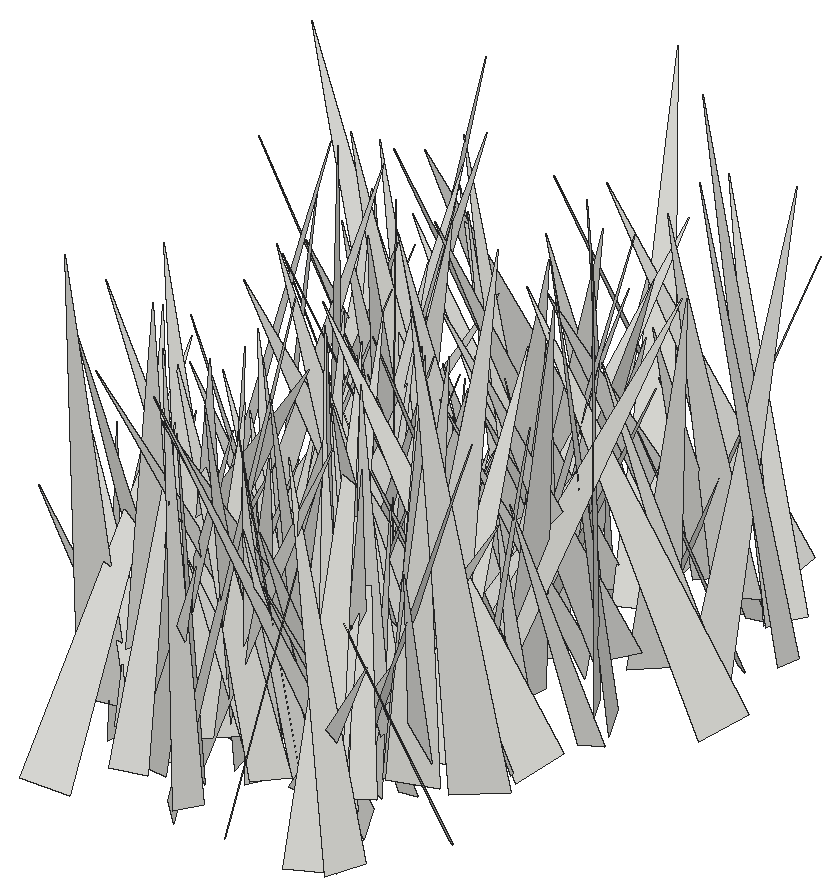
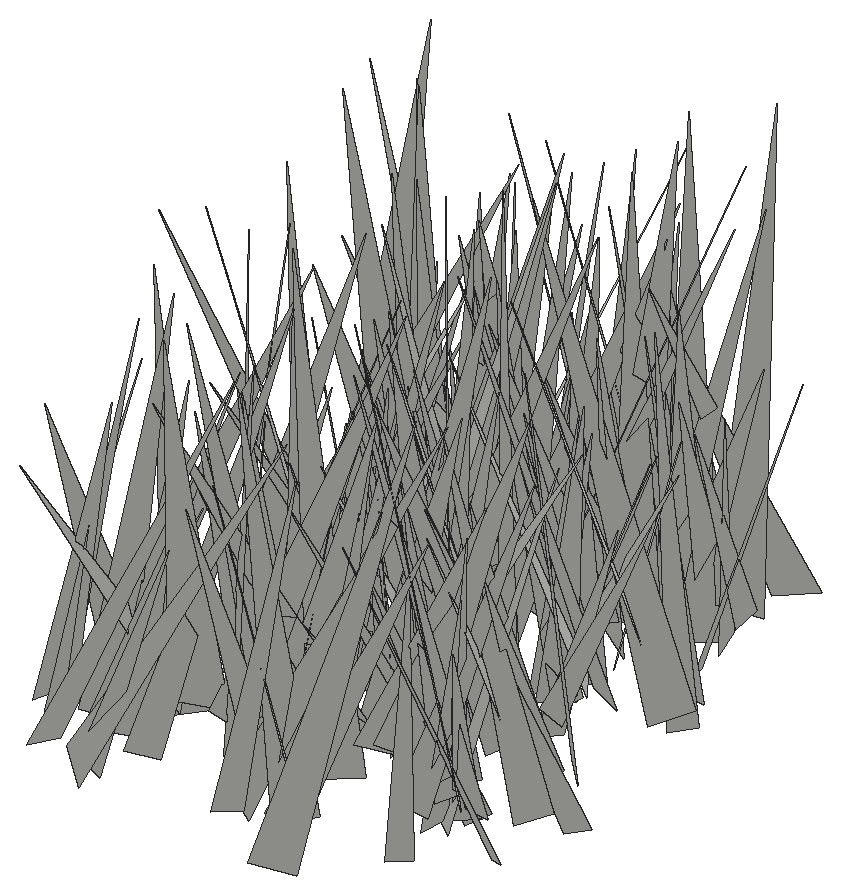
# SketchUp Ruby script. Lengths in inches.
U = 1.inch
M = Sketchup.active_model
def pt(a) = Geom::Point3d.new(a.map { |v| v * U })
def face(e, loops, mat)
  f = e.add_face(loops[0].map { |a| pt(a) })
  loops[1..].each { |l| e.add_face(l.map { |a| pt(a) }).erase! }
  f.material = f.back_material = mat if mat
  f
end
# faces: each face lists its corners as indices into pts; further lists are holes
def faces(e, pts, list, mat = nil) = list.each { |f| face(e, (f[0].is_a?(Array) ? f : [f]).map { |l| l.map { |i| pts[i] } }, mat) }
# xy, xz, yz: faces in a plane at the given z, y or x. An outline is a flat list of corners, or four numbers for a rectangle; further outlines are holes
def ring(l) = l.size == 4 ? [[l[0], l[1]], [l[2], l[1]], [l[2], l[3]], [l[0], l[3]]] : l.each_slice(2).to_a
def flat(e, list, mat, &to3) = list.each { |f| face(e, (f[0].is_a?(Array) ? f : [f]).map { |l| ring(l).map { |u, v| to3.(u, v) } }, mat) }
def xy(e, z, list, mat = nil) = flat(e, list, mat) { |x, y| [x, y, z] }
def xz(e, y, list, mat = nil) = flat(e, list, mat) { |x, z| [x, y, z] }
def yz(e, x, list, mat = nil) = flat(e, list, mat) { |y, z| [x, y, z] }
def lines(e, pts, list) = list.each { |a, b| e.add_line(pt(pts[a]), pt(pts[b])) }
# prism: a flat outline (further loops are holes) pulled along v
def prism(e, loops, v, mat = nil)
  f = face(e, loops, mat); d = Geom::Vector3d.new(v.map { |x| x * U })
  f.pushpull(f.normal.samedirection?(d) ? d.length : -d.length)
end
def box(e, o, s, mat = nil) = prism(e, [[o, [o[0] + s[0], o[1], o[2]], [o[0] + s[0], o[1] + s[1], o[2]], [o[0], o[1] + s[1], o[2]]]], [0, 0, s[2]], mat)
def at(x, y, z, deg = 0) = Geom::Transformation.translation(pt([x, y, z])) * Geom::Transformation.rotation(ORIGIN, Z_AXIS, deg.degrees)
def axes(o, x, y, z) = Geom::Transformation.new([*x, 0, *y, 0, *z, 0, *pt(o).to_a, 1])
def part(name) = M.definitions.add(name)
# library, detail: a bought-in or finely detailed component or shape, given as its bounding box
def library(name, o, s) = part(name).tap { |d| box(d.entities, o, s) }
def detail(e, o, s) = box(e.add_group.entities, o, s)
def put(e, d, t, mat = nil) = e.add_instance(d, t).tap { |i| i.material = mat if mat }
def group(e, t, mat = nil) = e.add_group.tap { |g| g.transformation = t; g.material = mat if mat }.entities
root = M.entities
c1 = part("fur_instance\#9")
p = [[0.8125,0,1.79],[0.67,-0.02,1.48],[0,-0.11,0],[0,0.11,0]]
faces(c1.entities,p,[[0,1,2,3]])
put(root,c1,axes([114.02,116.04,-27.1],[-0.24742,-3.68689,1.2628],[-3.55064,-0.30834,-1.59591],[-1.60648,1.24932,3.33279]))
put(root,c1,axes([111.5,119.83,-27.1],[4.04394,2.43918,0.42992],[2.39305,-4.06014,0.52577],[-0.63852,0.23141,4.69325]))
put(root,c1,axes([113.03,117.41,-28.22],[-4.3486,2.21974,0.80785],[1.83051,4.23636,-1.78683],[1.49303,1.27131,4.54366]))
put(root,c1,axes([113.39,120.65,-28.22],[-2.57238,2.98987,0.10946],[2.97729,2.57237,-0.29516],[0.29502,0.10983,3.93311]))
put(root,c1,axes([115.94,120.41,-27.1],[-4.22364,6.9226,0.63988],[6.72709,3.88063,2.42031],[-1.75445,-1.78585,7.73974]))
put(root,c1,axes([110.48,119.21,-28.22],[0.87918,5.14411,1.43079],[4.85097,-0.16366,-2.39235],[2.23095,-1.67133,4.63805]))
put(root,c1,axes([110.67,121.02,-27.1],[5.28357,-2.5058,0.04843],[-2.504,-5.27298,0.35108],[0.10676,0.33794,5.83712]))
put(root,c1,axes([113.7,121.4,-28.22],[-3.65311,-4.50937,0.62916],[-4.48426,3.70309,0.50402],[0.78847,0.16789,5.78149]))
put(root,c1,axes([113.92,121.53,-28.22],[-4.36363,0.98227,0.81119],[0.91976,4.432,-0.41906],[0.88144,0.23814,4.45315]))
put(root,c1,axes([113.81,122.78,-27.1],[0.77993,-5.26102,0.56712],[-5.12867,-0.89269,-1.22806],[-1.30258,0.36472,5.1748]))
put(root,c1,axes([114.15,120.3125,-27.1],[-5.02502,0.15502,0.9974],[-0.08895,4.97687,-1.22169],[1.00545,1.21508,4.87671]))
put(root,c1,axes([113.62,109.8,-28.22],[-4.09527,-2.1175,0.66115],[-1.87882,4.04889,1.32991],[1.17939,-0.90267,4.41434]))
put(root,c1,axes([113.2,108.08,-27.1],[-3.70619,1.07071,1.22273],[0.63141,3.75399,-1.37341],[1.4976,1.06701,3.605]))
put(root,c1,axes([112.73,116.55,-28.22],[4.54729,4.68314,2.12923],[4.88324,-4.82336,0.17985],[-1.61844,-1.39522,6.52513]))
put(root,c1,axes([114.97,115.28,-28.22],[-4.74174,-2.50609,0.51828],[-2.55748,4.67952,-0.77105],[0.09149,0.92453,5.30754]))
put(root,c1,axes([114.01,107.99,-28.22],[-4.48133,-0.60292,1.35721],[-0.97091,4.45413,-1.22715],[1.12377,1.44397,4.35201]))
put(root,c1,axes([114.64,115.36,-28.22],[-3.82314,1.91513,0.41484],[1.95484,3.79049,0.51675],[0.13566,-0.64863,4.24466]))
put(root,c1,axes([114.16,116.82,-28.22],[-5.42402,3.35952,0.54018],[3.08821,5.28712,-1.87283],[1.42868,1.32596,6.09909]))
put(root,c1,axes([116.91,119.8,-27.1],[-5.49378,-4.48735,0.1731],[-4.21573,5.05933,-2.64174],[-1.54724,2.14821,6.58325]))
put(root,c1,axes([111.83,112.71,-28.22],[5.73315,-1.08828,0.33068],[-0.98004,-5.58896,-1.40205],[-0.57725,-1.3198,5.66459]))
put(root,c1,axes([115.26,107.1,-27.1],[-5.60466,1.1961,0.32776],[0.92969,5.05609,-2.5538],[0.82084,2.4404,5.13039]))
put(root,c1,axes([111.19,122.08,-28.22],[3.29682,4.04593,0.27696],[3.82738,-2.98619,-1.93627],[1.34069,-1.42422,4.84659]))
put(root,c1,axes([115.87,107.25,-27.1],[-2.49681,4.68547,0.3153],[4.52882,2.308,1.56527],[-1.24213,-1.0033,5.07323]))
put(root,c1,axes([113.27,112.22,-27.1],[5.00071,5.94343,0.88428],[5.7504,-5.06729,1.53914],[-1.74336,0.3341,7.61331]))
put(root,c1,axes([113.77,107.82,-27.1],[1.30407,-7.61557,2.3618],[-7.95747,-1.39423,-0.10194],[-0.50366,2.30972,7.72574]))
put(root,c1,axes([114.55,112.42,-27.1],[-3.02688,-2.08558,0.64094],[-2.07151,3.09116,0.27563],[0.68504,0.13224,3.66547]))
put(root,c1,axes([115.68,113.24,-27.1],[-2.7303,-2.91554,0.15676],[-2.8364,2.59761,-1.08937],[-0.69267,0.85529,3.84294]))
put(root,c1,axes([116.74,120.65,-27.1],[-3.94655,4.7323,0.06828],[4.56087,3.77904,1.70056],[-1.26405,-1.13963,5.92267]))
put(root,c1,axes([112.63,111.09,-28.22],[-1.89095,-4.65132,2.366],[-4.60338,2.67208,1.57395],[2.45798,1.42605,4.76793]))
put(root,c1,axes([112.15,121.8,-27.1],[3.4737,5.90005,1.74495],[6.11319,-3.08303,-1.74525],[0.69596,-2.36778,6.62052]))
put(root,c1,axes([113.4,123.78,-28.22],[3.7269,-2.05729,0.24824],[-1.97365,-3.67974,-0.86491],[-0.63149,-0.64103,4.16823]))
put(root,c1,axes([113.13,121.38,-27.1],[5.7382,5.20942,1.87337],[5.41352,-5.84467,-0.3291],[-1.15821,-1.50876,7.74318]))
put(root,c1,axes([113.33,121.5625,-27.1],[4.73571,-1.08461,0.9225],[-1.0987,-4.82145,-0.02851],[-0.90568,0.17765,4.85824]))
put(root,c1,axes([114.72,127.98,-27.1],[4.75153,-4.99406,0.9078],[-4.47168,-4.70683,-2.48828],[-2.40183,-1.11663,6.42854]))
put(root,c1,axes([115.76,107.52,-28.22],[-5.08982,4.44528,0.70369],[4.40622,5.13821,-0.58816],[0.91699,-0.01575,6.73207]))
put(root,c1,axes([112.84,111.25,-28.22],[4.26787,-0.90452,0.30078],[-0.95208,-4.11231,1.14272],[-0.04649,1.18073,4.21035]))
put(root,c1,axes([115.4375,109.34,-27.1],[-1.29627,-6.42722,1.30707],[-6.54569,1.18361,-0.67151],[-0.41416,1.4099,6.52216]))
put(root,c1,axes([115.58,114.3,-28.22],[-4.07009,-1.55263,0.42821],[-1.43545,4.0247,0.94922],[0.73043,-0.7422,4.25151]))
put(root,c1,axes([114.27,104.43,-28.22],[-2.48989,6.58556,0.19317],[6.42005,2.47161,-1.51018],[1.47984,0.3578,6.87667]))
put(root,c1,axes([115.29,120.33,-28.22],[0.65749,-6.30029,1.7132],[-6.47052,-0.85883,-0.67511],[-0.87239,1.62165,6.29842]))
put(root,c1,axes([113.45,114.24,-27.1],[3.5873,6.66463,1.07182],[6.75002,-3.55215,-0.50434],[-0.05834,-1.18311,7.55193]))
put(root,c1,axes([115.72,113.67,-28.22],[3.17127,-3.30736,3.04126],[-3.82504,-3.9403,-0.2965],[-2.35731,1.94429,4.57249]))
put(root,c1,axes([113.14,120.47,-28.22],[2.74116,-2.85153,0.16279],[-2.64199,-2.44575,1.64616],[1.08517,1.2485,3.59657]))
put(root,c1,axes([117.54,123.87,-28.22],[-4.20776,3.77593,1.0344],[3.85861,3.7428,2.0336],[-0.66241,-2.18328,5.27517]))
put(root,c1,axes([113.4,118.2,-27.1],[4.3525,2.53578,0.43229],[2.57081,-4.2585,-0.90411],[0.08934,-0.99816,4.9555]))
put(root,c1,axes([115.15,116.42,-28.22],[-5.30404,4.85737,1.41696],[4.30663,5.41145,-2.42976],[2.65607,0.92563,6.76928]))
put(root,c1,axes([111.27,113.91,-27.1],[2.01455,-7.63294,0.11302],[-6.59973,-1.68273,3.99311],[3.83642,1.11337,6.80994]))
put(root,c1,axes([116.54,113.45,-28.22],[-5.03296,-0.41167,1.23228],[-0.52474,5.15421,-0.42127],[1.18855,0.5323,5.03216]))
put(root,c1,axes([116.49,113.04,-28.22],[-3.50037,2.65675,1.28484],[2.86731,3.53339,0.50538],[0.69832,-1.19104,4.36526]))
put(root,c1,axes([114.875,108.5,-28.22],[4.71718,-6.41333,2.08506],[-6.64537,-4.85367,0.10513],[-1.14777,1.74389,7.96063]))
put(root,c1,axes([116.49,110.02,-28.22],[2.34142,5.16985,1.64131],[5.10687,-2.70355,1.23051],[-1.82787,-0.93109,5.54034]))
put(root,c1,axes([114.38,113.92,-27.1],[4.71146,3.59222,0.48874],[3.58656,-4.73541,0.23065],[-0.52868,-0.11206,5.92019]))
put(root,c1,axes([119.03,108.63,-27.1],[-7.40149,0.22253,0.007],[0.22253,7.40149,0.00759],[0.00677,-0.0078,7.40483]))
put(root,c1,axes([115.52,108.19,-28.22],[4.65785,-0.69082,1.21899],[-0.53967,-4.78978,-0.65231],[-1.29303,-0.48941,4.6634]))
put(root,c1,axes([119.43,116.89,-28.22],[-0.98442,7.82804,0.7856],[7.24103,0.59195,3.17514],[-3.07617,-1.11168,7.22258]))
put(root,c1,axes([119.22,123.96,-28.22],[-3.5976,-6.50533,0.64098],[-6.34012,3.29439,-2.15004],[-1.59153,1.58132,7.11613]))
put(root,c1,axes([117.55,108.19,-27.1],[3.71191,-5.65782,4.04126],[-6.28277,-4.69165,-0.79764],[-2.97818,2.84578,6.7196]))
put(root,c1,axes([118.01,118.71,-28.22],[-4.3642,6.37446,3.0679],[7.06974,4.05938,1.62241],[0.25406,-3.46117,7.553]))
put(root,c1,axes([116.57,109.33,-27.1],[-1.7521,4.37342,1.24469],[4.49457,1.86786,-0.23622],[0.6891,-1.06311,4.7054]))
put(root,c1,axes([116.49,114.98,-27.1],[7.01213,2.59998,3.36264],[2.81322,-7.70163,0.08845],[-3.18638,-1.07803,7.47811]))
put(root,c1,axes([115.33,113.61,-28.22],[4.85484,-0.93426,0.93937],[-1.01134,-4.91828,0.33525],[-0.85583,0.51221,4.93253]))
put(root,c1,axes([119.17,120.8,-28.22],[-6.47288,0.26814,0.01301],[0.25719,6.28405,-1.55397],[0.07694,1.55212,6.2893]))
put(root,c1,axes([116.85,105.0625,-27.1],[-1.85743,4.94831,0.92273],[4.99711,1.93095,-0.29602],[0.60509,-0.75691,5.27714]))
put(root,c1,axes([115.04,119.2,-28.22],[4.2743,-5.66959,1.70794],[-5.91958,-4.14155,1.06631],[-0.14077,2.00854,7.01974]))
put(root,c1,axes([116.39,111.77,-27.1],[-0.0874,4.08723,0.80677],[4.1529,0.14964,-0.30818],[0.33125,-0.79758,4.07653]))
put(root,c1,axes([115.93,115.375,-28.22],[5.15399,5.0376,1.12923],[4.93282,-5.27609,1.02292],[-1.5231,-0.04087,7.13405]))
put(root,c1,axes([115.65,110.125,-27.1],[5.14782,-4.26055,1.16689],[-4.27581,-5.25589,-0.32723],[-1.10966,0.4872,6.67423]))
put(root,c1,axes([115.52,119.42,-28.22],[7.57168,-2.77915,1.4038],[-2.39268,-7.55557,-2.05259],[-1.99233,-1.48808,7.80006]))
put(root,c1,axes([116.4,115.59,-27.1],[-0.03084,5.75903,1.17934],[5.85206,0.14189,-0.53988],[0.55736,-1.17118,5.73375]))
put(root,c1,axes([118.19,111.2,-27.1],[-6.16351,-3.9605,0.27898],[-3.73191,5.95492,2.08903],[1.35509,-1.6142,7.02213]))
put(root,c1,axes([116.01,109.52,-27.1],[4.17653,-0.25853,0.87813],[-0.4857,-4.1025,1.10224],[-0.77592,1.17643,4.03674]))
put(root,c1,axes([114.96,109.01,-27.1],[3.94876,4.2171,2.00571],[4.64379,-3.26946,-2.26834],[0.4919,-2.98768,5.31331]))
put(root,c1,axes([117.28,107.8,-28.22],[-3.42106,-4.15596,2.05732],[-4.44833,3.66341,0.00339],[1.31032,1.58608,5.3829]))
put(root,c1,axes([115.7,112.32,-28.22],[4.00821,-3.73033,0.31245],[-3.73197,-4.01777,-0.09299],[-0.29215,0.14465,5.47471]))
put(root,c1,axes([116.73,116.02,-28.22],[-0.99114,4.85366,1.48422],[5.00835,1.18049,-0.51592],[0.82303,-1.33855,4.92689]))
put(root,c1,axes([118.53,120.74,-27.1],[-5.56537,0.35389,1.01892],[0.25962,5.63719,-0.53984],[1.04691,0.48332,5.55042]))
put(root,c1,axes([118.12,112.79,-28.22],[0.5097,3.85536,0.87755],[3.83119,-0.70034,0.85159],[-0.9777,-0.73445,3.79452]))
put(root,c1,axes([118.95,116.91,-28.22],[-7.12654,1.94071,2.81889],[3.04033,6.57978,3.15641],[1.57127,-3.9294,6.67765]))
put(root,c1,axes([116.65,110.62,-27.1],[5.33264,0.16428,1.51785],[-0.27785,-5.31816,1.55174],[-1.50122,1.56784,5.10452]))
put(root,c1,axes([115.97,107.14,-28.22],[1.4923,-4.43759,0.64343],[-4.35505,-1.27294,1.3215],[1.06759,1.01025,4.49142]))
put(root,c1,axes([119.5,104.49,-27.1],[-6.71,0.21588,0.88951],[-0.0468,6.49159,-1.92847],[0.91413,1.91692,6.43053]))
put(root,c1,axes([116.26,116.11,-27.1],[4.91416,0.05831,0.74386],[0.02898,-4.96646,0.19783],[-0.74558,0.19125,4.91052]))
put(root,c1,axes([117.86,126.13,-27.1],[-4.50462,1.14541,2.32905],[1.86637,4.67145,1.31236],[1.80364,-1.97324,4.45884]))
put(root,c1,axes([117.9,118.83,-27.1],[-4.53794,-6.8341,0.16977],[-6.57814,4.42074,2.12406],[1.86058,-1.03861,7.92377]))
put(root,c1,axes([119.57,115.48,-28.22],[-5.44212,1.96061,0.21811],[1.90755,5.39324,-0.88463],[0.50284,0.7598,5.71648]))
put(root,c1,axes([120.79,119.32,-28.22],[-0.71343,7.62578,1.29035],[7.14993,0.15622,3.02994],[-2.94889,-1.46615,7.03427]))
put(root,c1,axes([116.5,118.18,-28.22],[1.15422,4.7345,0.08294],[4.6056,-1.10261,-1.15208],[1.10037,-0.35121,4.73502]))
put(root,c1,axes([119.75,123.21,-28.22],[-5.4355,-1.48683,0.1699],[-1.41481,5.31415,1.24191],[0.48767,-1.15472,5.49664]))
put(root,c1,axes([117.7,118.57,-28.22],[3.13173,2.6382,1.54856],[2.8558,-3.31576,-0.12654],[-1.0966,-1.10068,4.0929]))
put(root,c1,axes([120.31,107.28,-27.1],[-1.88222,6.06948,1.49765],[6.0067,1.32242,2.18977],[-1.73238,-2.00921,5.96542]))
put(root,c1,axes([119.08,112.77,-28.22],[2.70234,-6.75975,0.1599],[-6.39067,-2.60962,-2.31767],[-2.20886,-0.71979,6.90111]))
put(root,c1,axes([117.62,109.67,-28.22],[6.82649,-0.20783,2.36031],[0.47416,-6.93274,-1.9818],[-2.32152,-2.02711,6.5358]))
put(root,c1,axes([116.67,124.43,-27.1],[3.8282,2.91024,0.83789],[3.01788,-3.55309,-1.44728],[0.25298,-1.65308,4.58585]))
put(root,c1,axes([118.45,115.14,-28.22],[-5.8561,-4.67693,3.47291],[-5.12361,6.47844,0.0849],[2.77191,2.09401,7.49403]))
put(root,c1,axes([119.16,110.6875,-27.1],[-5.25856,3.05312,1.43062],[2.8843,5.44607,-1.02073],[1.74617,0.1987,5.99435]))
put(root,c1,axes([118.02,105.54,-28.22],[-5.10797,-4.03263,5.02727],[-5.71036,5.80586,-1.14484],[2.98787,4.202,6.40647]))
put(root,c1,axes([118.54,121.07,-28.22],[4.42124,-3.27,0.9733],[-2.9097,-4.44582,-1.71927],[-1.78153,-0.85401,5.22344]))
put(root,c1,axes([117.18,123.82,-28.22],[5.59181,-3.37862,1.09906],[-3.46581,-5.63815,0.30113],[-0.78177,0.82912,6.52631]))
put(root,c1,axes([118.41,117.47,-28.22],[2.33806,3.32528,1.40975],[3.5899,-2.32407,-0.47188],[-0.3968,-1.43269,4.03749]))
put(root,c1,axes([117.76,118.71,-28.22],[-0.58442,-4.16845,1.10453],[-3.96593,0.95723,1.51414],[1.69333,0.80327,3.92746]))
put(root,c1,axes([118.97,108.74,-28.22],[4.37094,-3.26497,1.75227],[-3.26747,-4.6741,-0.55863],[-1.74761,0.57306,5.42707]))
put(root,c1,axes([120.86,113.01,-27.1],[-6.83352,3.26319,2.339],[3.80782,6.73136,1.73366],[1.27275,-2.61852,7.37155]))
put(root,c1,axes([119.63,121.39,-28.22],[-3.40624,-2.616,1.08161],[-2.59295,3.56228,0.44999],[1.13575,0.28715,4.27123]))
put(root,c1,axes([118.52,115.86,-27.1],[3.43862,2.40363,0.16823],[2.31203,-3.37399,0.94893],[-0.67841,0.6845,4.08669]))
put(root,c1,axes([120.89,117.54,-28.22],[-7.26017,0.65472,1.63239],[0.85,7.37598,0.82207],[1.53976,-0.9847,7.24313]))
put(root,c1,axes([120.97,122.09,-27.1],[0.32689,-6.93131,1.01824],[-6.72809,-0.59471,-1.88835],[-1.95261,0.88881,6.67713]))
put(root,c1,axes([119.48,122.62,-27.1],[4.39596,-0.31282,2.17467],[-1.10489,-4.51925,1.5834],[-1.89902,1.90528,4.11281]))
put(root,c1,axes([116.32,108.73,-28.22],[5.46808,5.3055,1.78388],[5.41419,-4.38056,-3.56761],[1.42026,-3.72732,6.73205]))
put(root,c1,axes([117.07,114.49,-28.22],[6.89965,2.05968,0.48381],[2.11498,-6.67017,-1.76557],[0.05673,-1.82978,6.98071]))
put(root,c1,axes([118.375,115.58,-27.1],[4.08731,-3.32744,0.79787],[-3.41978,-4.01464,0.77613],[-0.11643,1.10699,5.21302]))
put(root,c1,axes([120.05,109.89,-28.22],[-1.31696,-6.51866,1.83434],[-6.75362,1.40125,0.13086],[0.49623,1.77078,6.64907]))
put(root,c1,axes([117.81,121.11,-28.22],[3.30529,-7.09092,0.75642],[-7.06387,-3.14139,1.41833],[0.97724,1.27626,7.69379]))
put(root,c1,axes([120.51,108.27,-27.1],[-3.95359,-4.39819,1.62013],[-4.4402,4.19331,0.54823],[1.50116,0.81969,5.8885]))
put(root,c1,axes([119.1875,113.97,-27.1],[4.30125,1.72732,0.68489],[1.69718,-4.35514,0.32517],[-0.75649,0.05042,4.6237]))
put(root,c1,axes([120.65,122.59,-28.22],[-4.32305,-4.69404,2.5219],[-5.10648,4.57733,-0.23372],[1.52244,2.02405,6.37716]))
put(root,c1,axes([122.9,108.55,-28.22],[-6.73685,-3.71008,0.0403],[-3.70619,6.73292,0.28887],[0.17463,-0.23362,7.68547]))
put(root,c1,axes([119.25,114.35,-28.22],[2.10072,-7.09935,0.00934],[-7.09522,-2.09917,0.25546],[0.24231,0.08144,7.39923]))
put(root,c1,axes([120.81,109.71,-28.22],[4.24793,5.0228,3.04998],[5.34423,-4.86703,0.57187],[-2.44337,-1.91294,6.55335]))
put(root,c1,axes([118.97,118.86,-28.22],[-0.93463,7.10607,0.24964],[6.82555,0.96718,-1.97702],[1.99262,0.02006,6.88921]))
put(root,c1,axes([121.07,108.36,-28.22],[-4.57691,0.82768,1.57562],[1.18388,4.66198,0.99001],[1.32893,-1.30255,4.54457]))
put(root,c1,axes([120.98,121.58,-28.22],[0.9036,-5.03288,0.01557],[-4.93923,-0.88981,-0.97923],[-0.96652,-0.158,5.01871]))
put(root,c1,axes([119.79,114.99,-27.1],[-0.91828,3.53646,1.4047],[3.57282,1.29857,-0.93362],[1.30946,-1.06309,3.53244]))
put(root,c1,axes([121.59,115.89,-28.22],[-3.92471,-3.72483,0.22437],[-3.66233,3.90735,0.80501],[0.71557,-0.43166,5.35067]))
put(root,c1,axes([123.21,115.39,-27.1],[-3.40667,-4.88664,0.79026],[-4.79108,3.01371,-2.01797],[-1.2447,1.77411,5.60468]))
put(root,c1,axes([124.19,125.3,-28.22],[-4.6508,-5.63712,0.37429],[-5.36466,4.25457,-2.58191],[-1.77136,1.91537,6.83673]))
put(root,c1,axes([119.92,105.75,-28.22],[3.92442,2.27765,0.90763],[2.32456,-4.0011,-0.01041],[-0.77966,-0.46478,4.53747]))
put(root,c1,axes([122.9,107.1,-28.22],[-7.30125,2.0292,0.54339],[1.84392,7.1322,-1.85816],[1.00641,1.65384,7.34664]))
put(root,c1,axes([122.38,121.79,-27.1],[-3.14428,7.71271,0.49149],[7.72648,3.12546,0.38342],[-0.17032,-0.59964,8.32018]))
put(root,c1,axes([122.17,107.06,-28.22],[-0.64935,7.68845,0.01437],[7.6155,0.6412,1.06165],[-1.05669,-0.10353,7.64243]))
put(root,c1,axes([119.46,120.41,-28.22],[3.73697,-5.4189,0.58942],[-5.45085,-3.71358,0.41766],[0.01126,0.72231,6.56925]))
put(root,c1,axes([121.36,116.3,-28.22],[-2.17037,-5.72704,0.1674],[-5.69455,2.17595,0.61228],[0.63178,-0.0613,6.09382]))
put(root,c1,axes([120.91,110.24,-28.22],[1.9027,-5.40071,0.1352],[-5.35593,-1.9045,-0.70218],[-0.70705,-0.10684,5.68285]))
put(root,c1,axes([119.25,122.73,-27.1],[4.36325,-2.68491,0.18726],[-2.69098,-4.34538,0.39756],[0.04948,0.43666,5.1077]))
put(root,c1,axes([121.86,111.09,-27.1],[-3.05036,2.77962,1.08054],[2.93347,3.07501,0.37088],[0.53722,-1.00823,4.11016]))
put(root,c1,axes([121.81,114.84,-28.22],[-4.33048,1.8912,1.2808],[1.94847,4.49129,-0.04381],[1.19187,-0.47097,4.72523]))
put(root,c1,axes([121.28,116.19,-27.1],[1.03899,3.82207,0.22987],[3.79032,-1.06041,0.49963],[-0.54276,-0.08876,3.92914]))
put(root,c1,axes([118.87,122.33,-27.1],[6.16535,-1.94029,0.16764],[-1.94054,-6.16752,-0.01601],[-0.16472,0.03505,6.46343]))
put(root,c1,axes([121.3125,110.71,-28.22],[-3.6044,-3.37024,0.34721],[-3.01204,3.4196,1.92476],[1.55135,-1.19103,4.54373]))
put(root,c1,axes([122.98,107.9375,-27.1],[-0.78819,5.89997,0.04998],[5.7265,0.75282,1.4401],[-1.42105,-0.23877,5.77555]))
put(root,c1,axes([121.59,110.375,-27.1],[-0.9402,5.50023,2.63792],[6.09336,0.97222,0.14463],[0.28664,-2.62629,5.57814]))
put(root,c1,axes([120.83,121.84,-27.1],[-2.98653,-2.99705,1.42564],[-2.58075,3.30304,1.53746],[2.08674,-0.20437,3.94181]))
put(root,c1,axes([120.87,110.35,-28.22],[5.28351,-1.61661,1.62366],[-1.56193,-5.52709,-0.42043],[-1.67632,0.05465,5.50927]))
put(root,c1,axes([120.57,119.72,-28.22],[4.80209,-1.99507,1.20954],[-2.10711,-4.89697,0.2883],[-1.00169,0.73669,5.19204]))
put(root,c1,axes([121.875,110.11,-28.22],[1.76175,3.91399,1.38102],[4.01071,-1.99148,0.5277],[-1.06803,-1.02224,4.25965]))
put(root,c1,axes([123.31,105.32,-28.22],[-6.67493,4.02137,0.12146],[3.83511,6.43107,-2.16198],[1.21576,1.79188,7.48679]))
put(root,c1,axes([121.8,125.1,-27.1],[6.11084,-2.63091,1.80363],[-1.49433,-5.80472,-3.40432],[-2.81811,-2.62692,5.71618]))
put(root,c1,axes([120.39,118.64,-28.22],[4.79219,0.94532,0.41054],[0.81575,-4.67249,1.23678],[-0.62985,1.14081,4.72537]))
put(root,c1,axes([122.68,110.63,-28.22],[-0.75955,-3.70224,0.74684],[-3.72635,0.61048,-0.76351],[-0.61539,0.87293,3.70143]))
put(root,c1,axes([124.53,126.23,-27.1],[-6.85321,0.30824,0.48855],[0.41589,6.6696,1.62593],[0.40091,-1.64973,6.66467]))
put(root,c1,axes([121.11,112.84,-27.1],[0.6303,-6.24139,2.24897],[-6.57772,-0.29373,1.02832],[0.86396,2.31708,6.18828]))
put(root,c1,axes([120.21,115.72,-27.1],[1.05381,5.0713,0.10966],[4.76326,-0.95083,-1.80217],[1.74396,-0.4674,4.856]))
put(root,c1,axes([123.16,118.29,-27.1],[-4.86193,-2.9811,0.43497],[-2.74592,4.72474,1.68858],[1.2394,-1.22654,5.44739]))
put(root,c1,axes([123.82,125.05,-28.22],[-1.05055,-3.99645,1.56356],[-4.12582,0.49771,-1.49997],[-1.18067,1.81677,3.85037]))
put(root,c1,axes([124.06,106.03,-28.22],[-5.92125,2.00992,1.02968],[2.02644,6.00419,-0.06686],[0.99676,-0.26678,6.25272]))
put(root,c1,axes([125.47,112.06,-27.1],[-5.46904,-3.01802,0.13387],[-2.92547,5.22183,-1.79189],[-0.75368,1.63119,5.98398]))
put(root,c1,axes([122.93,115.66,-28.22],[0.17752,-3.57602,1.3313],[-3.7929,-0.31113,-0.32997],[-0.41733,1.30655,3.56518]))
put(root,c1,axes([125.95,112.62,-27.1],[-7.5943,2.08618,0.38061],[2.11361,7.33132,1.9887],[-0.17228,-2.01745,7.62041]))
put(root,c1,axes([123.13,110.98,-27.1],[-3.56356,5.20391,0.71647],[5.00613,3.62664,-1.4419],[1.59144,0.24443,6.14008]))
put(root,c1,axes([124.14,124.89,-28.22],[-0.63614,-4.28295,0.71253],[-4.25699,0.4736,-0.95381],[-0.85404,0.8295,4.22357]))
put(root,c1,axes([122.86,124.46,-27.1],[2.86729,-4.50295,0.62999],[-4.43501,-2.93396,-0.78577],[-1.00209,0.10064,5.2802]))
put(root,c1,axes([121.77,116.21,-27.1],[5.53821,4.98185,1.27941],[5.04776,-5.62536,0.05401],[-0.98782,-0.81487,7.449]))
put(root,c1,axes([123.64,119.1,-27.1],[3.27903,-5.74844,0.73311],[-5.41958,-3.34021,-1.9507],[-2.05188,-0.36394,6.32387]))
put(root,c1,axes([122.41,111.9,-27.1],[-3.47776,6.78239,3.15196],[7.08859,4.09761,-0.99596],[2.38486,-2.28893,7.55669]))
put(root,c1,axes([121.49,107.21,-27.1],[1.52564,-3.34819,0.07276],[-3.07421,-1.36842,1.48995],[1.32851,0.67846,3.36423]))
put(root,c1,axes([121.82,116.97,-28.22],[7.47084,-2.00529,1.5784],[-1.88161,-7.62701,-0.78379],[-1.72397,-0.36551,7.69548]))
put(root,c1,axes([123.08,113.17,-28.22],[3.52114,3.87417,1.40413],[3.91467,-3.72163,0.45161],[-1.28689,-0.72073,5.21571]))
put(root,c1,axes([125.4,109.19,-28.22],[-2.7685,-2.84273,0.0732],[-2.6967,2.59213,-1.32656],[-0.90237,0.97511,3.73978]))
put(root,c1,axes([122.8125,110.22,-27.1],[7.01983,-0.71592,2.31882],[-0.6287,-7.39114,-0.37866],[-2.34397,-0.1616,7.04608]))
put(root,c1,axes([120.91,110.31,-27.1],[4.20762,-3.32651,0.12048],[-3.15177,-3.91891,1.86887],[1.07075,1.53645,5.02763]))
put(root,c1,axes([125.91,123.75,-27.1],[-7.81157,-0.92448,1.21309],[-1.13809,7.74743,-1.42443],[1.01538,1.5715,7.73604]))
put(root,c1,axes([124.1,124.01,-27.1],[1.75802,-6.33898,1.96931],[-6.51413,-2.03906,-0.74828],[-1.27556,1.67662,6.53555]))
put(root,c1,axes([123.1,121.625,-27.1],[4.98815,3.01806,0.37753],[2.59556,-4.60182,2.49383],[-1.58564,1.9615,5.26983]))
put(root,c1,axes([124.7,117.57,-28.22],[-6.35073,-3.49942,2.22612],[-3.7296,6.59945,-0.26567],[1.81428,1.31702,7.24617]))
put(root,c1,axes([120.93,115.32,-28.22],[1.74287,7.71217,1.36191],[7.45298,-1.20484,-2.71503],[2.4053,-1.85492,7.42588]))
put(root,c1,axes([123.65,109.62,-27.1],[-2.45983,6.23998,3.07468],[6.83629,2.77173,-0.15592],[1.28687,-2.79677,6.7055]))
put(root,c1,axes([126.08,123.78,-27.1],[-6.2227,2.39174,0.32304],[2.36421,6.22042,-0.51348],[0.48507,0.36431,6.64671]))
put(root,c1,axes([123.68,110.03,-27.1],[0.0585,-4.06465,0.78718],[-4.11626,0.02739,0.44734],[0.44434,0.78888,4.04038]))
put(root,c1,axes([125.57,122.36,-28.22],[-2.53875,-3.10556,0.31926],[-3.0835,2.42999,-0.88252],[-0.48832,0.80145,3.91291]))
put(root,c1,axes([120.82,110.67,-28.22],[8.07507,1.50255,0.4439],[1.56674,-7.73574,-2.31627],[0.00564,-2.35841,7.88031]))
put(root,c1,axes([125.01,116.14,-28.22],[0.25989,-4.12749,1.06746],[-4.12688,-0.51192,-0.97467],[-1.06982,0.97209,4.01917]))
put(root,c1,axes([125.03,116.38,-27.1],[-5.7993,-3.05465,2.69516],[-3.68736,5.92923,-1.21419],[1.7315,2.39584,6.44116]))
put(root,c1,axes([127.35,119.33,-28.22],[-6.93796,2.79801,1.11968],[3.01121,6.55067,2.28891],[0.12298,-2.54512,7.12215]))
put(root,c1,axes([123.57,120.79,-28.22],[5.17414,-4.36417,1.70527],[-4.54977,-5.28673,0.27499],[-1.1196,1.31532,6.76329]))
put(root,c1,axes([125.83,120.39,-28.22],[-7.01528,2.7432,0.95764],[2.14491,6.5776,-3.12905],[1.96,2.6204,6.85188]))
put(root,c1,axes([126.63,120.05,-28.22],[-5.6933,-0.47947,0.5538],[-0.44449,5.71072,0.37467],[0.58224,-0.32872,5.70116]))
put(root,c1,axes([125.53,110.38,-27.1],[3.59874,-6.83955,3.08177],[-7.12327,-4.18751,-0.97538],[-2.35281,2.21652,7.66674]))
put(root,c1,axes([127.67,121.9,-27.1],[-6.96753,-1.64469,0.65915],[-1.76863,6.61713,-2.18437],[0.10697,2.27915,6.81763]))
